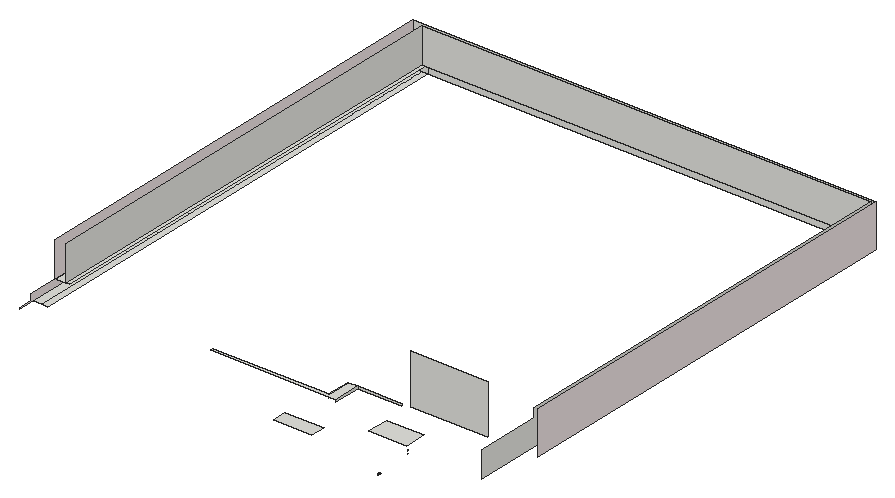
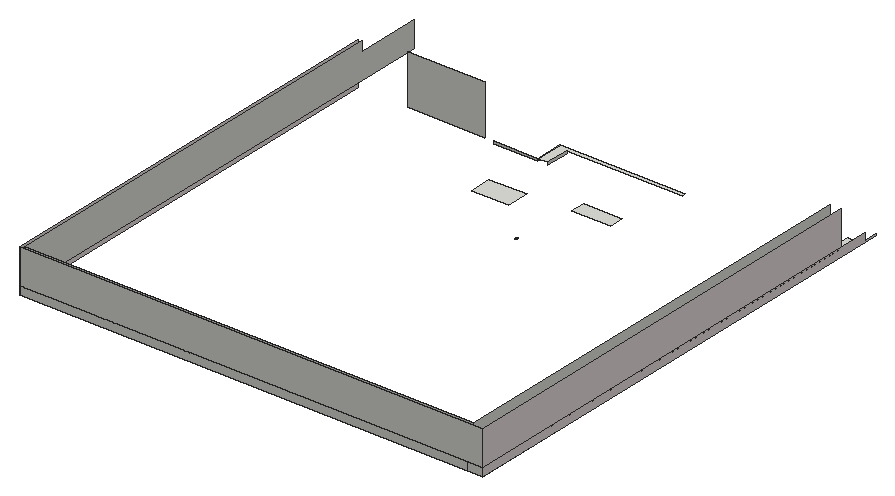
# SketchUp Ruby script. Lengths in inches.
U = 1.inch
M = Sketchup.active_model
def pt(a) = Geom::Point3d.new(a.map { |v| v * U })
def face(e, loops, mat)
  f = e.add_face(loops[0].map { |a| pt(a) })
  loops[1..].each { |l| e.add_face(l.map { |a| pt(a) }).erase! }
  f.material = f.back_material = mat if mat
  f
end
# faces: each face lists its corners as indices into pts; further lists are holes
def faces(e, pts, list, mat = nil) = list.each { |f| face(e, (f[0].is_a?(Array) ? f : [f]).map { |l| l.map { |i| pts[i] } }, mat) }
# xy, xz, yz: faces in a plane at the given z, y or x. An outline is a flat list of corners, or four numbers for a rectangle; further outlines are holes
def ring(l) = l.size == 4 ? [[l[0], l[1]], [l[2], l[1]], [l[2], l[3]], [l[0], l[3]]] : l.each_slice(2).to_a
def flat(e, list, mat, &to3) = list.each { |f| face(e, (f[0].is_a?(Array) ? f : [f]).map { |l| ring(l).map { |u, v| to3.(u, v) } }, mat) }
def xy(e, z, list, mat = nil) = flat(e, list, mat) { |x, y| [x, y, z] }
def xz(e, y, list, mat = nil) = flat(e, list, mat) { |x, z| [x, y, z] }
def yz(e, x, list, mat = nil) = flat(e, list, mat) { |y, z| [x, y, z] }
def lines(e, pts, list) = list.each { |a, b| e.add_line(pt(pts[a]), pt(pts[b])) }
# prism: a flat outline (further loops are holes) pulled along v
def prism(e, loops, v, mat = nil)
  f = face(e, loops, mat); d = Geom::Vector3d.new(v.map { |x| x * U })
  f.pushpull(f.normal.samedirection?(d) ? d.length : -d.length)
end
def box(e, o, s, mat = nil) = prism(e, [[o, [o[0] + s[0], o[1], o[2]], [o[0] + s[0], o[1] + s[1], o[2]], [o[0], o[1] + s[1], o[2]]]], [0, 0, s[2]], mat)
def at(x, y, z, deg = 0) = Geom::Transformation.translation(pt([x, y, z])) * Geom::Transformation.rotation(ORIGIN, Z_AXIS, deg.degrees)
def axes(o, x, y, z) = Geom::Transformation.new([*x, 0, *y, 0, *z, 0, *pt(o).to_a, 1])
def part(name) = M.definitions.add(name)
# library, detail: a bought-in or finely detailed component or shape, given as its bounding box
def library(name, o, s) = part(name).tap { |d| box(d.entities, o, s) }
def detail(e, o, s) = box(e.add_group.entities, o, s)
def put(e, d, t, mat = nil) = e.add_instance(d, t).tap { |i| i.material = mat if mat }
def group(e, t, mat = nil) = e.add_group.tap { |g| g.transformation = t; g.material = mat if mat }.entities
root = M.entities
M.materials.add("Generic\#9").color = [233, 223, 223]
M.materials.add("Material \#1").color = [140, 140, 140]
xy(root,194.16,[[388.01,199.78,387.96,199.8,387.97,199.81],[388.01,199.78,387.97,199.81,388.02,199.79],[388.01,199.78,388.02,199.79,388.07,199.78],[388.07,199.78,388.02,199.79,388.07,199.79],[388.07,199.78,388.07,199.79,388.13,199.8],
  [388.07,199.79,388.12,199.81,388.13,199.8],[387.96,199.8,387.91,199.83,387.92,199.84],[387.96,199.8,387.92,199.84,387.97,199.81],[388.13,199.8,388.12,199.81,388.18,199.83],[388.12,199.81,388.16,199.84,388.18,199.83],
  [387.91,199.83,387.88,199.88,387.9,199.88],[387.91,199.83,387.9,199.88,387.92,199.84],[388.18,199.83,388.16,199.84,388.21,199.88],[388.16,199.84,388.19,199.88,388.21,199.88],[387.88,199.88,387.87,199.93,387.89,199.93],
  [387.88,199.88,387.89,199.93,387.9,199.88],[388.19,199.88,388.2,199.93,388.22,199.93],[388.19,199.88,388.22,199.93,388.21,199.88],[387.87,199.93,387.88,199.98,387.9,199.98],[387.87,199.93,387.9,199.98,387.89,199.93],
  [388.2,199.93,388.19,199.98,388.21,199.98],[388.2,199.93,388.21,199.98,388.22,199.93],[387.88,199.98,387.91,200.03,387.92,200.02],[387.88,199.98,387.92,200.02,387.9,199.98],[388.19,199.98,388.16,200.02,388.18,200.03],
  [388.19,199.98,388.18,200.03,388.21,199.98],[387.92,200.02,387.91,200.03,387.97,200.05],[388.16,200.02,388.12,200.05,388.13,200.07],[388.16,200.02,388.13,200.07,388.18,200.03],[387.91,200.03,387.96,200.07,387.97,200.05],
  [387.97,200.05,387.96,200.07,388.02,200.07],[388.12,200.05,388.07,200.07,388.07,200.08],[388.12,200.05,388.07,200.08,388.13,200.07],[387.96,200.07,388.01,200.08,388.02,200.07],[388.02,200.07,388.01,200.08,388.07,200.07],
  [388.07,200.07,388.01,200.08,388.07,200.08]],"Material \#1")
xy(root,194.18,[[388.01,199.78,388.02,199.79,387.96,199.8],[388.01,199.78,388.07,199.78,388.07,199.79],[388.01,199.78,388.07,199.79,388.02,199.79],[388.07,199.78,388.12,199.81,388.07,199.79],[388.07,199.78,388.13,199.8,388.12,199.81],
  [388.02,199.79,387.97,199.81,387.96,199.8],[387.96,199.8,387.97,199.81,387.91,199.83],[388.13,199.8,388.16,199.84,388.12,199.81],[388.13,199.8,388.18,199.83,388.16,199.84],[387.97,199.81,387.92,199.84,387.91,199.83],
  [387.91,199.83,387.92,199.84,387.88,199.88],[388.18,199.83,388.19,199.88,388.16,199.84],[388.18,199.83,388.21,199.88,388.19,199.88],[387.92,199.84,387.9,199.88,387.88,199.88],[387.88,199.88,387.9,199.88,387.87,199.93],
  [387.9,199.88,387.89,199.93,387.87,199.93],[388.19,199.88,388.21,199.88,388.2,199.93],[388.21,199.88,388.22,199.93,388.2,199.93],[387.87,199.93,387.89,199.93,387.88,199.98],[387.89,199.93,387.9,199.98,387.88,199.98],
  [388.2,199.93,388.22,199.93,388.19,199.98],[388.22,199.93,388.21,199.98,388.19,199.98],[387.88,199.98,387.9,199.98,387.91,200.03],[387.9,199.98,387.92,200.02,387.91,200.03],[388.19,199.98,388.21,199.98,388.16,200.02],
  [388.21,199.98,388.18,200.03,388.16,200.02],[387.92,200.02,387.96,200.07,387.91,200.03],[387.92,200.02,387.97,200.05,387.96,200.07],[388.16,200.02,388.18,200.03,388.12,200.05],[388.18,200.03,388.13,200.07,388.12,200.05],
  [387.97,200.05,388.01,200.08,387.96,200.07],[387.97,200.05,388.02,200.07,388.01,200.08],[388.12,200.05,388.13,200.07,388.07,200.07],[388.02,200.07,388.07,200.08,388.01,200.08],[388.02,200.07,388.07,200.07,388.07,200.08],
  [388.07,200.07,388.13,200.07,388.07,200.08]],"Material \#1")
xy(root,197.47,[[388.01,199.78,387.96,199.8,388.02,199.79],[388.01,199.78,388.02,199.79,388.07,199.79],[388.01,199.78,388.07,199.79,388.07,199.78],[388.07,199.78,388.07,199.79,388.12,199.81],[388.07,199.78,388.12,199.81,388.13,199.8],
  [388.02,199.79,387.96,199.8,387.97,199.81],[387.96,199.8,387.91,199.83,387.97,199.81],[388.13,199.8,388.12,199.81,388.16,199.84],[388.13,199.8,388.16,199.84,388.18,199.83],[387.97,199.81,387.91,199.83,387.92,199.84],
  [387.91,199.83,387.88,199.88,387.92,199.84],[388.18,199.83,388.16,199.84,388.19,199.88],[388.18,199.83,388.19,199.88,388.21,199.88],[387.92,199.84,387.88,199.88,387.9,199.88],[387.88,199.88,387.87,199.93,387.9,199.88],
  [387.9,199.88,387.87,199.93,387.89,199.93],[388.19,199.88,388.2,199.93,388.21,199.88],[388.21,199.88,388.2,199.93,388.22,199.93],[387.87,199.93,387.88,199.98,387.89,199.93],[387.89,199.93,387.88,199.98,387.9,199.98],
  [388.2,199.93,388.19,199.98,388.22,199.93],[388.22,199.93,388.19,199.98,388.21,199.98],[387.88,199.98,387.91,200.03,387.9,199.98],[387.9,199.98,387.91,200.03,387.92,200.02],[388.19,199.98,388.16,200.02,388.21,199.98],
  [388.21,199.98,388.16,200.02,388.18,200.03],[387.92,200.02,387.91,200.03,387.96,200.07],[387.92,200.02,387.96,200.07,387.97,200.05],[388.16,200.02,388.12,200.05,388.18,200.03],[388.18,200.03,388.12,200.05,388.13,200.07],
  [387.97,200.05,387.96,200.07,388.01,200.08],[387.97,200.05,388.01,200.08,388.02,200.07],[388.12,200.05,388.07,200.07,388.13,200.07],[388.02,200.07,388.01,200.08,388.07,200.08],[388.02,200.07,388.07,200.08,388.07,200.07],
  [388.07,200.07,388.07,200.08,388.13,200.07]],"Material \#1")
xy(root,197.49,[[388.01,199.78,387.97,199.81,387.96,199.8],[388.01,199.78,388.02,199.79,387.97,199.81],[388.01,199.78,388.07,199.78,388.02,199.79],[388.07,199.78,388.07,199.79,388.02,199.79],[388.07,199.78,388.13,199.8,388.07,199.79],
  [388.07,199.79,388.13,199.8,388.12,199.81],[387.96,199.8,387.92,199.84,387.91,199.83],[387.96,199.8,387.97,199.81,387.92,199.84],[388.13,199.8,388.18,199.83,388.12,199.81],[388.12,199.81,388.18,199.83,388.16,199.84],
  [387.91,199.83,387.9,199.88,387.88,199.88],[387.91,199.83,387.92,199.84,387.9,199.88],[388.18,199.83,388.21,199.88,388.16,199.84],[388.16,199.84,388.21,199.88,388.19,199.88],[387.88,199.88,387.89,199.93,387.87,199.93],
  [387.88,199.88,387.9,199.88,387.89,199.93],[388.19,199.88,388.21,199.88,388.22,199.93],[388.19,199.88,388.22,199.93,388.2,199.93],[387.87,199.93,387.89,199.93,387.9,199.98],[387.87,199.93,387.9,199.98,387.88,199.98],
  [388.2,199.93,388.21,199.98,388.19,199.98],[388.2,199.93,388.22,199.93,388.21,199.98],[387.88,199.98,387.9,199.98,387.92,200.02],[387.88,199.98,387.92,200.02,387.91,200.03],[388.19,199.98,388.18,200.03,388.16,200.02],
  [388.19,199.98,388.21,199.98,388.18,200.03],[387.92,200.02,387.97,200.05,387.91,200.03],[388.16,200.02,388.13,200.07,388.12,200.05],[388.16,200.02,388.18,200.03,388.13,200.07],[387.91,200.03,387.97,200.05,387.96,200.07],
  [387.97,200.05,388.02,200.07,387.96,200.07],[388.12,200.05,388.07,200.08,388.07,200.07],[388.12,200.05,388.13,200.07,388.07,200.08],[387.96,200.07,388.02,200.07,388.01,200.08],[388.02,200.07,388.07,200.07,388.01,200.08],
  [388.07,200.07,388.07,200.08,388.01,200.08]],"Material \#1")
xy(root,198.6875,[[279.74,171.4375,317.36,185.375]])
xy(root,204.625,[[354.24,194.75,390.67,216.25]])
xy(root,240,[[67.11,143.9375,75.375,607.4375],[75.375,143.9375,80.9375,607.4375],[220.54,168.26,220.54,171.4375,333.65,171.4375,333.65,194.75,342.98,194.75,342.98,168.26]])
xy(root,247.625,[[67.11,170.6875,77.5625,170.6875,77.5625,605.125,80.9375,605.125,80.9375,607.4375,67.11,607.4375],[77.5625,170.6875,80.9375,605.125]])
xz(root,194.75,[[342.98,237.6875,385.91,240],[394.85,240,470.29,288.79]])
xz(root,199.31,[[358.95,166.41,358.96,166.53,358.96,166.41],[358.96,166.41,358.96,166.53,358.97,166.53],[360.15,166.41,360.14,166.53,360.16,166.41],[360.16,166.41,360.14,166.53,360.15,166.53],[359.52,166.46,359.48,166.47,359.52,166.47],
  [359.52,166.46,359.52,166.47,359.55,166.47],[359.52,166.46,359.55,166.47,359.55,166.46],[359.55,166.46,359.55,166.47,359.59,166.47],[359.55,166.46,359.59,166.47,359.59,166.46],[359.59,166.46,359.59,166.47,359.62,166.48],
  [359.59,166.46,359.62,166.48,359.62,166.47],[359.48,166.47,359.45,166.49,359.48,166.48],[359.48,166.47,359.48,166.48,359.52,166.47],[359.62,166.47,359.62,166.48,359.65,166.5],[359.62,166.47,359.65,166.5,359.65,166.49],
  [359.48,166.48,359.45,166.49,359.46,166.5],[359.45,166.49,359.42,166.51,359.46,166.5],[359.65,166.49,359.65,166.5,359.67,166.52],[359.65,166.49,359.67,166.52,359.68,166.51],[359.46,166.5,359.42,166.51,359.43,166.52],
  [359.42,166.51,359.4,166.53,359.43,166.52],[359.68,166.51,359.67,166.52,359.7,166.54],[359.68,166.51,359.7,166.54,359.7,166.53],[359.43,166.52,359.4,166.53,359.41,166.54],[358.96,166.53,358.98,166.64,358.97,166.53],
  [358.97,166.53,358.98,166.64,358.99,166.63],[359.4,166.53,359.38,166.5625,359.41,166.54],[359.7,166.53,359.7,166.54,359.72,166.57],[359.7,166.53,359.72,166.57,359.72,166.5625],[360.14,166.53,360.11,166.63,360.15,166.53],
  [360.15,166.53,360.11,166.63,360.12,166.64],[359.41,166.54,359.38,166.5625,359.39,166.57],[359.38,166.5625,359.36,166.6,359.39,166.57],[359.72,166.5625,359.72,166.57,359.73,166.6],[359.72,166.5625,359.73,166.6,359.74,166.6],
  [359.39,166.57,359.36,166.6,359.37,166.6],[359.36,166.6,359.35,166.63,359.37,166.6],[359.37,166.6,359.35,166.63,359.36,166.64],[359.73,166.6,359.74,166.64,359.74,166.6],[359.74,166.6,359.74,166.64,359.75,166.63],
  [358.99,166.63,358.98,166.64,359.03,166.74],[358.99,166.63,359.03,166.74,359.04,166.73],[359.35,166.63,359.35,166.68,359.36,166.64],[359.75,166.63,359.74,166.64,359.74,166.67],[359.75,166.63,359.74,166.67,359.75,166.67],
  [360.11,166.63,360.0625,166.73,360.12,166.64],[359.36,166.64,359.35,166.68,359.36,166.68],[360.12,166.64,360.0625,166.73,360.07,166.74],[359.74,166.67,359.74,166.71,359.75,166.67],[359.75,166.67,359.74,166.71,359.75,166.71],
  [359.35,166.68,359.35,166.71,359.36,166.68],[359.36,166.68,359.35,166.71,359.36,166.71],[359.35,166.71,359.36,166.75,359.36,166.71],[359.36,166.71,359.36,166.75,359.37,166.74],[359.74,166.71,359.73,166.74,359.75,166.71],
  [359.75,166.71,359.73,166.74,359.74,166.75],[359.04,166.73,359.03,166.74,359.09,166.83],[359.04,166.73,359.09,166.83,359.1,166.82],[360.0625,166.73,360.01,166.82,360.07,166.74],[359.37,166.74,359.36,166.75,359.38,166.78],
  [359.37,166.74,359.38,166.78,359.39,166.77],[359.73,166.74,359.72,166.77,359.74,166.75],[360.07,166.74,360.01,166.82,360.01,166.83],[359.74,166.75,359.72,166.77,359.72,166.78],[359.39,166.77,359.38,166.78,359.4,166.81],
  [359.39,166.77,359.4,166.81,359.41,166.8],[359.72,166.77,359.7,166.8,359.72,166.78],[359.72,166.78,359.7,166.8,359.7,166.81],[359.41,166.8,359.4,166.81,359.42,166.84],[359.41,166.8,359.42,166.84,359.43,166.83],
  [359.7,166.8,359.67,166.83,359.7,166.81],[359.7,166.81,359.67,166.83,359.68,166.84],[359.1,166.82,359.09,166.83,359.16,166.91],[359.1,166.82,359.16,166.91,359.17,166.9],[360.01,166.82,359.93,166.9,360.01,166.83],
  [359.43,166.83,359.42,166.84,359.45,166.86],[359.43,166.83,359.45,166.86,359.46,166.85],[359.67,166.83,359.65,166.85,359.68,166.84],[360.01,166.83,359.93,166.9,359.94,166.91],[359.68,166.84,359.65,166.85,359.65,166.86],
  [359.46,166.85,359.45,166.86,359.48,166.87],[359.46,166.85,359.48,166.87,359.48,166.86],[359.65,166.85,359.62,166.86,359.65,166.86],[359.48,166.86,359.48,166.87,359.52,166.88],[359.48,166.86,359.52,166.88,359.52,166.87],
  [359.62,166.86,359.59,166.87,359.62,166.87],[359.62,166.86,359.62,166.87,359.65,166.86],[359.52,166.87,359.52,166.88,359.55,166.89],[359.52,166.87,359.55,166.89,359.55,166.875],[359.59,166.87,359.55,166.875,359.59,166.88],
  [359.59,166.87,359.59,166.88,359.62,166.87],[359.55,166.875,359.55,166.89,359.59,166.88],[359.17,166.9,359.16,166.91,359.25,166.97],[359.17,166.9,359.25,166.97,359.25,166.96],[359.93,166.9,359.85,166.96,359.94,166.91],
  [359.94,166.91,359.85,166.96,359.86,166.97],[359.25,166.96,359.25,166.97,359.34,167.02],[359.25,166.96,359.34,167.02,359.34,167.01],[359.85,166.96,359.76,167.01,359.86,166.97],[359.86,166.97,359.76,167.01,359.76,167.02],
  [359.34,167.01,359.34,167.02,359.44,167.05],[359.34,167.01,359.44,167.05,359.44,167.04],[359.76,167.01,359.66,167.04,359.76,167.02],[359.76,167.02,359.66,167.04,359.66,167.05],[359.44,167.04,359.44,167.05,359.55,167.06],
  [359.44,167.04,359.55,167.06,359.55,167.05],[359.66,167.04,359.55,167.05,359.66,167.05],[359.55,167.05,359.55,167.06,359.66,167.05]],"Material \#1")
xz(root,201.11,[[358.95,166.41,358.96,166.41,358.96,166.53],[358.96,166.41,358.97,166.53,358.96,166.53],[360.15,166.41,360.16,166.41,360.14,166.53],[360.16,166.41,360.15,166.53,360.14,166.53],[359.52,166.46,359.52,166.47,359.48,166.47],
  [359.52,166.46,359.55,166.46,359.55,166.47],[359.52,166.46,359.55,166.47,359.52,166.47],[359.55,166.46,359.59,166.46,359.59,166.47],[359.55,166.46,359.59,166.47,359.55,166.47],[359.59,166.46,359.62,166.47,359.62,166.48],
  [359.59,166.46,359.62,166.48,359.59,166.47],[359.48,166.47,359.48,166.48,359.45,166.49],[359.48,166.47,359.52,166.47,359.48,166.48],[359.62,166.47,359.65,166.49,359.65,166.5],[359.62,166.47,359.65,166.5,359.62,166.48],
  [359.48,166.48,359.46,166.5,359.45,166.49],[359.45,166.49,359.46,166.5,359.42,166.51],[359.65,166.49,359.67,166.52,359.65,166.5],[359.65,166.49,359.68,166.51,359.67,166.52],[359.46,166.5,359.43,166.52,359.42,166.51],
  [359.42,166.51,359.43,166.52,359.4,166.53],[359.68,166.51,359.7,166.54,359.67,166.52],[359.68,166.51,359.7,166.53,359.7,166.54],[359.43,166.52,359.41,166.54,359.4,166.53],[358.96,166.53,358.97,166.53,358.98,166.64],
  [358.97,166.53,358.99,166.63,358.98,166.64],[359.4,166.53,359.41,166.54,359.38,166.5625],[359.7,166.53,359.72,166.5625,359.72,166.57],[359.7,166.53,359.72,166.57,359.7,166.54],[360.14,166.53,360.15,166.53,360.11,166.63],
  [360.15,166.53,360.12,166.64,360.11,166.63],[359.41,166.54,359.39,166.57,359.38,166.5625],[359.38,166.5625,359.39,166.57,359.36,166.6],[359.72,166.5625,359.73,166.6,359.72,166.57],[359.72,166.5625,359.74,166.6,359.73,166.6],
  [359.39,166.57,359.37,166.6,359.36,166.6],[359.36,166.6,359.37,166.6,359.35,166.63],[359.37,166.6,359.36,166.64,359.35,166.63],[359.73,166.6,359.74,166.6,359.74,166.64],[359.74,166.6,359.75,166.63,359.74,166.64],
  [358.99,166.63,359.03,166.74,358.98,166.64],[358.99,166.63,359.04,166.73,359.03,166.74],[359.35,166.63,359.36,166.64,359.35,166.68],[359.75,166.63,359.74,166.67,359.74,166.64],[359.75,166.63,359.75,166.67,359.74,166.67],
  [360.11,166.63,360.12,166.64,360.0625,166.73],[359.36,166.64,359.36,166.68,359.35,166.68],[360.12,166.64,360.07,166.74,360.0625,166.73],[359.74,166.67,359.75,166.67,359.74,166.71],[359.75,166.67,359.75,166.71,359.74,166.71],
  [359.35,166.68,359.36,166.68,359.35,166.71],[359.36,166.68,359.36,166.71,359.35,166.71],[359.35,166.71,359.36,166.71,359.36,166.75],[359.36,166.71,359.37,166.74,359.36,166.75],[359.74,166.71,359.75,166.71,359.73,166.74],
  [359.75,166.71,359.74,166.75,359.73,166.74],[359.04,166.73,359.09,166.83,359.03,166.74],[359.04,166.73,359.1,166.82,359.09,166.83],[360.0625,166.73,360.07,166.74,360.01,166.82],[359.37,166.74,359.38,166.78,359.36,166.75],
  [359.37,166.74,359.39,166.77,359.38,166.78],[359.73,166.74,359.74,166.75,359.72,166.77],[360.07,166.74,360.01,166.83,360.01,166.82],[359.74,166.75,359.72,166.78,359.72,166.77],[359.39,166.77,359.4,166.81,359.38,166.78],
  [359.39,166.77,359.41,166.8,359.4,166.81],[359.72,166.77,359.72,166.78,359.7,166.8],[359.72,166.78,359.7,166.81,359.7,166.8],[359.41,166.8,359.42,166.84,359.4,166.81],[359.41,166.8,359.43,166.83,359.42,166.84],
  [359.7,166.8,359.7,166.81,359.67,166.83],[359.7,166.81,359.68,166.84,359.67,166.83],[359.1,166.82,359.16,166.91,359.09,166.83],[359.1,166.82,359.17,166.9,359.16,166.91],[360.01,166.82,360.01,166.83,359.93,166.9],
  [359.43,166.83,359.45,166.86,359.42,166.84],[359.43,166.83,359.46,166.85,359.45,166.86],[359.67,166.83,359.68,166.84,359.65,166.85],[360.01,166.83,359.94,166.91,359.93,166.9],[359.68,166.84,359.65,166.86,359.65,166.85],
  [359.46,166.85,359.48,166.87,359.45,166.86],[359.46,166.85,359.48,166.86,359.48,166.87],[359.65,166.85,359.65,166.86,359.62,166.86],[359.48,166.86,359.52,166.87,359.52,166.88],[359.48,166.86,359.52,166.88,359.48,166.87],
  [359.62,166.86,359.62,166.87,359.59,166.87],[359.62,166.86,359.65,166.86,359.62,166.87],[359.52,166.87,359.55,166.875,359.55,166.89],[359.52,166.87,359.55,166.89,359.52,166.88],[359.59,166.87,359.59,166.88,359.55,166.875],
  [359.59,166.87,359.62,166.87,359.59,166.88],[359.55,166.875,359.59,166.88,359.55,166.89],[359.17,166.9,359.25,166.97,359.16,166.91],[359.17,166.9,359.25,166.96,359.25,166.97],[359.93,166.9,359.94,166.91,359.85,166.96],
  [359.94,166.91,359.86,166.97,359.85,166.96],[359.25,166.96,359.34,167.01,359.34,167.02],[359.25,166.96,359.34,167.02,359.25,166.97],[359.85,166.96,359.86,166.97,359.76,167.01],[359.86,166.97,359.76,167.02,359.76,167.01],
  [359.34,167.01,359.44,167.04,359.44,167.05],[359.34,167.01,359.44,167.05,359.34,167.02],[359.76,167.01,359.76,167.02,359.66,167.04],[359.76,167.02,359.66,167.05,359.66,167.04],[359.44,167.04,359.55,167.05,359.55,167.06],
  [359.44,167.04,359.55,167.06,359.44,167.05],[359.66,167.04,359.66,167.05,359.55,167.05],[359.55,167.05,359.66,167.05,359.55,167.06]],"Material \#1")
xz(root,605.125,[[77.5625,247.625,515.25,281.9]])
xz(root,607.4375,[[67.11,240,80.9375,247.625],[80.9375,240,518.6875,247.625],[67.11,247.625,518.6875,281.9]])
yz(root,67.11,[[127.4375,240,127.4375,241.3125,140.625,241.3125,140.625,247.625,607.4375,247.625,607.4375,240],[170.6875,247.625,170.6875,271.31,170.75,271.31,170.75,274.25,170.6875,274.25,170.6875,281.9,607.4375,281.9,607.4375,247.625]],"Generic\#9")
yz(root,77.5625,[[170.6875,247.625,605.125,281.9]])
yz(root,333.65,[[171.4375,237.1875,194.75,240]])
yz(root,342.98,[[168.26,237.6875,194.75,240]])
yz(root,515.25,[[131.45,247.625,131.45,272.4375,194.75,272.4375,194.75,281.9,605.125,281.9,605.125,247.625]])
yz(root,518.6875,[[194.75,240,607.4375,281.9]],"Generic\#9")
p = [[359.5,199.31,166.72],[359.5,199.33,166.72],[359.5625,199.33,166.6],[359.5625,199.31,166.6],[359.6,199.31,166.625],[359.6,199.33,166.625],
  [359.54,199.33,166.74],[359.54,199.31,166.74],[359.57,199.33,166.58],[359.57,199.31,166.58],[359.59,199.34,166.55],[359.59,199.31,166.55],
  [359.61,199.34,166.5625],[359.61,199.31,166.5625],[359.63,199.34,166.58],[359.63,199.31,166.58],[359.62,199.33,166.6],[359.62,199.31,166.6],
  [359.5,201.12,166.72],[359.5625,201.12,166.6],[359.5625,201.09,166.6],[359.5,201.09,166.72],[359.6,201.12,166.625],[359.54,201.12,166.74],
  [359.54,201.09,166.74],[359.6,201.09,166.625],[359.57,201.11,166.58],[359.57,201.09,166.58],[359.59,201.11,166.55],[359.59,201.08,166.55],
  [359.61,201.11,166.5625],[359.61,201.08,166.5625],[359.63,201.11,166.58],[359.63,201.08,166.58],[359.62,201.11,166.6],[359.62,201.09,166.6],
  [359.53,199.33,166.76],[359.53,199.31,166.76],[359.47,199.31,166.76],[359.47,199.34,166.76],[359.49,199.33,166.74],[359.49,199.31,166.74],
  [359.53,201.11,166.76],[359.53,201.09,166.76],[359.47,201.11,166.76],[359.49,201.11,166.74],[359.49,201.09,166.74],[359.47,201.08,166.76],
  [359.51,199.34,166.79],[359.51,199.31,166.79],[359.49,199.34,166.78],[359.49,199.31,166.78],[359.51,201.11,166.79],[359.51,201.08,166.79],
  [359.49,201.11,166.78],[359.49,201.08,166.78]]
faces(root,p,[[0,1,2],[2,3,0],[4,5,6],[6,7,4],[3,2,8],[8,9,3],[9,8,10],[10,11,9],
  [11,10,12],[12,13,11],[13,12,14],[14,15,13],[15,14,16],[16,17,15],[17,16,5],[5,4,17],
  [18,19,20],[20,21,18],[22,23,24],[24,25,22],[19,26,27],[27,20,19],[26,28,29],[29,27,26],
  [28,30,31],[31,29,28],[30,32,33],[33,31,30],[32,34,35],[35,33,32],[34,22,25],[25,35,34],
  [7,6,36],[36,37,7],[38,39,40],[40,41,38],[41,40,1],[1,0,41],[23,42,43],[43,24,23],
  [44,45,46],[46,47,44],[45,18,21],[21,46,45],[37,36,48],[48,49,37],[49,48,50],[50,51,49],
  [51,50,39],[39,38,51],[42,52,53],[53,43,42],[52,54,55],[55,53,52],[54,44,47],[47,55,54]],"Material \#1")
